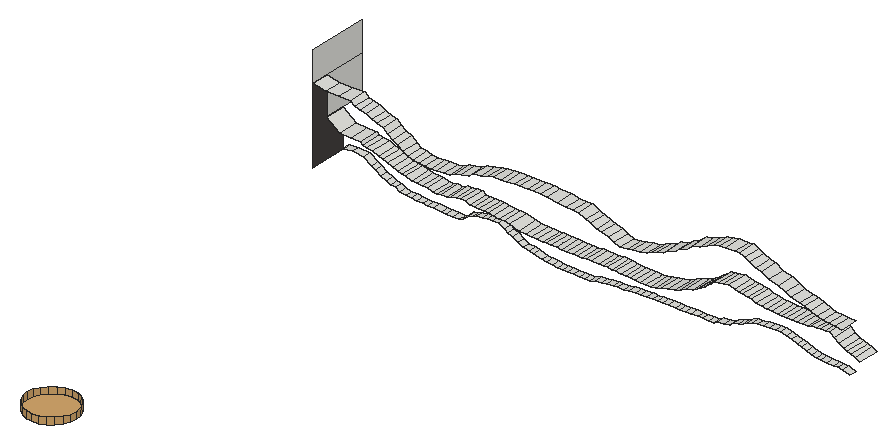
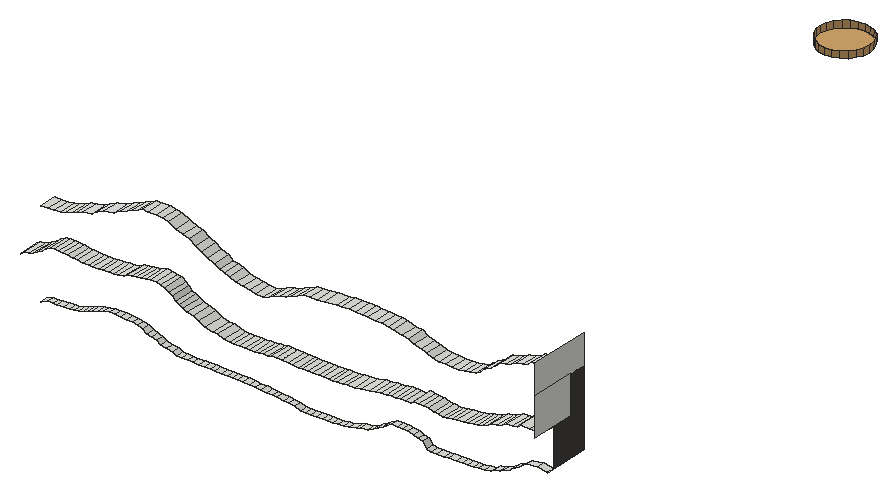
# SketchUp Ruby script. Lengths in inches.
U = 1.inch
M = Sketchup.active_model
def pt(a) = Geom::Point3d.new(a.map { |v| v * U })
def face(e, loops, mat)
  f = e.add_face(loops[0].map { |a| pt(a) })
  loops[1..].each { |l| e.add_face(l.map { |a| pt(a) }).erase! }
  f.material = f.back_material = mat if mat
  f
end
# faces: each face lists its corners as indices into pts; further lists are holes
def faces(e, pts, list, mat = nil) = list.each { |f| face(e, (f[0].is_a?(Array) ? f : [f]).map { |l| l.map { |i| pts[i] } }, mat) }
# xy, xz, yz: faces in a plane at the given z, y or x. An outline is a flat list of corners, or four numbers for a rectangle; further outlines are holes
def ring(l) = l.size == 4 ? [[l[0], l[1]], [l[2], l[1]], [l[2], l[3]], [l[0], l[3]]] : l.each_slice(2).to_a
def flat(e, list, mat, &to3) = list.each { |f| face(e, (f[0].is_a?(Array) ? f : [f]).map { |l| ring(l).map { |u, v| to3.(u, v) } }, mat) }
def xy(e, z, list, mat = nil) = flat(e, list, mat) { |x, y| [x, y, z] }
def xz(e, y, list, mat = nil) = flat(e, list, mat) { |x, z| [x, y, z] }
def yz(e, x, list, mat = nil) = flat(e, list, mat) { |y, z| [x, y, z] }
def lines(e, pts, list) = list.each { |a, b| e.add_line(pt(pts[a]), pt(pts[b])) }
# prism: a flat outline (further loops are holes) pulled along v
def prism(e, loops, v, mat = nil)
  f = face(e, loops, mat); d = Geom::Vector3d.new(v.map { |x| x * U })
  f.pushpull(f.normal.samedirection?(d) ? d.length : -d.length)
end
def box(e, o, s, mat = nil) = prism(e, [[o, [o[0] + s[0], o[1], o[2]], [o[0] + s[0], o[1] + s[1], o[2]], [o[0], o[1] + s[1], o[2]]]], [0, 0, s[2]], mat)
def at(x, y, z, deg = 0) = Geom::Transformation.translation(pt([x, y, z])) * Geom::Transformation.rotation(ORIGIN, Z_AXIS, deg.degrees)
def axes(o, x, y, z) = Geom::Transformation.new([*x, 0, *y, 0, *z, 0, *pt(o).to_a, 1])
def part(name) = M.definitions.add(name)
# library, detail: a bought-in or finely detailed component or shape, given as its bounding box
def library(name, o, s) = part(name).tap { |d| box(d.entities, o, s) }
def detail(e, o, s) = box(e.add_group.entities, o, s)
def put(e, d, t, mat = nil) = e.add_instance(d, t).tap { |i| i.material = mat if mat }
def group(e, t, mat = nil) = e.add_group.tap { |g| g.transformation = t; g.material = mat if mat }.entities
root = M.entities
M.materials.add("[Field Square Tile]").color = [211, 167, 108]
M.materials.add("[Granite Tile]1").color = [68, 65, 63]
xy(root,237.65,[[2918.33,565.74,2919.02,566.68],[2919.02,565.74,2919.64,566.68]])
xy(root,238.33,[[2927.43,565.74,2927.98,566.68],[2927.98,565.74,2928.66,566.68]])
xy(root,238.34,[[2929.34,565.74,2930.27,566.68],[2930.27,565.74,2930.76,566.68],[2930.76,565.74,2931.52,566.68],[2931.52,565.74,2932.15,566.68],[2932.15,565.74,2932.9,566.68],
  [2932.9,565.74,2933.52,566.68],[2933.52,565.74,2934.29,566.68],[2934.29,565.74,2934.91,566.68]])
xy(root,241.52,[[2889.03,561.05,2889.09,566.68]])
xy(root,241.68,[[2919.53,563.18,2920.12,565.74]])
xy(root,241.75,[[2921.88,563.18,2922.75,565.74],[2922.75,563.18,2923.37,565.74],[2923.37,563.18,2923.88,565.74]])
xy(root,250.6875,[[2909.35,492.27,2908.56,492.375,2907.82,492.68,2907.18,493.17,2906.7,493.8,2906.39,494.54,2906.29,495.33,2906.39,496.125,2906.7,496.86,2907.18,497.5,2907.82,497.98,2908.56,498.29,2909.35,498.39,2910.14,498.29,2910.88,497.98,2911.51,497.5,2912,496.86,2912.31,496.125,2912.41,495.33,2912.31,494.54,2912,493.8,2911.51,493.17,2910.88,492.68,2910.14,492.375]],"[Field Square Tile]")
xz(root,561.05,[[2889.03,241.52,2889.09,251.5]])
yz(root,2889.09,[[563.18,246.2,568.68,250.88],[561.05,250.88,568.68,254.5]])
yz(root,2889.09,[[561.05,241.52,565.74,241.52,565.74,246.2,563.18,246.2,563.18,250.88,561.05,250.88]],"[Granite Tile]1")
p = [[2919.64,565.74,237.65],[2919.64,566.68,237.65],[2920.31,566.68,237.89],[2920.31,565.74,237.89],[2914.97,565.74,237.76],[2914.97,566.68,237.76],
  [2915.68,566.68,237.71],[2915.68,565.74,237.71],[2916.29,566.68,237.68],[2916.29,565.74,237.68],[2916.89,566.68,237.67],[2916.89,565.74,237.67],
  [2917.64,566.68,237.66],[2917.64,565.74,237.66],[2918.33,566.68,237.65],[2918.33,565.74,237.65],[2913.62,565.74,237.9],[2913.62,566.68,237.9],
  [2914.28,566.68,237.82],[2914.28,565.74,237.82],[2912.68,565.74,238.21],[2912.68,566.68,238.21],[2921.07,566.68,237.94],[2921.07,565.74,237.94],
  [2921.6875,566.68,237.98],[2921.6875,565.74,237.98],[2922.54,566.68,238.1],[2922.54,565.74,238.1],[2923.09,566.68,238.13],[2923.09,565.74,238.13],
  [2923.85,566.68,238.15],[2923.85,565.74,238.15],[2912.21,565.74,238.31],[2912.21,566.68,238.31],[2924.48,566.68,238.26],[2924.48,565.74,238.26],
  [2911.3,565.74,238.43],[2911.3,566.68,238.43],[2925.23,566.68,238.28],[2925.23,565.74,238.28],[2925.86,566.68,238.3],[2925.86,565.74,238.3],
  [2926.71,566.68,238.32],[2926.71,565.74,238.32],[2927.43,566.68,238.33],[2927.43,565.74,238.33],[2928.66,565.74,238.33],[2928.66,566.68,238.33],
  [2929.34,566.68,238.34],[2929.34,565.74,238.34],[2934.91,565.74,238.34],[2934.91,566.68,238.34],[2935.42,566.68,238.59],[2935.42,565.74,238.59],
  [2910.65,565.74,238.74],[2910.65,566.68,238.74],[2950.94,565.74,238.78],[2950.94,566.68,238.78],[2951.72,566.68,238.43],[2951.72,565.74,238.43],
  [2936.24,566.68,238.72],[2936.24,565.74,238.72],[2910.07,565.74,239.11],[2910.07,566.68,239.11],[2936.93,566.68,238.86],[2936.93,565.74,238.86],
  [2900.28,565.74,238.92],[2900.28,566.68,238.92],[2901.32,566.68,238.82],[2901.32,565.74,238.82],[2901.83,566.68,238.8],[2901.83,565.74,238.8],
  [2902.7,566.68,238.79],[2902.7,565.74,238.79],[2903.44,566.68,238.77],[2903.44,565.74,238.77],[2903.97,566.68,238.9375],[2903.97,565.74,238.9375],
  [2948.22,565.74,238.875],[2948.22,566.68,238.875],[2948.97,566.68,238.83],[2948.97,565.74,238.83],[2949.73,566.68,238.8],[2949.73,565.74,238.8],
  [2950.27,566.68,238.79],[2950.27,565.74,238.79],[2898.19,565.74,238.97],[2898.19,566.68,238.97],[2898.89,566.68,238.94],[2898.89,565.74,238.94],
  [2899.59,566.68,238.93],[2899.59,565.74,238.93],[2904.53,566.68,239.55],[2904.53,565.74,239.55],[2937.44,566.68,239.18],[2937.44,565.74,239.18],
  [2947.07,565.74,239.04],[2947.07,566.68,239.04],[2947.65,566.68,238.94],[2947.65,565.74,238.94],[2896.82,565.74,239.09],[2896.82,566.68,239.09],
  [2897.51,566.68,239.03],[2897.51,565.74,239.03],[2946.41,565.74,239.29],[2946.41,566.68,239.29],[2896.04,565.74,239.19],[2896.04,566.68,239.19],
  [2909.49,565.74,239.38],[2909.49,566.68,239.38],[2895.53,565.74,239.52],[2895.53,566.68,239.52],[2938.03,566.68,239.35],[2938.03,565.74,239.35],
  [2945.83,565.74,239.53],[2945.83,566.68,239.53],[2909.03,565.74,239.71],[2909.03,566.68,239.71],[2938.59,566.68,239.52],[2938.59,565.74,239.52],
  [2894.97,565.74,239.64],[2894.97,566.68,239.64],[2939.14,566.68,239.85],[2939.14,565.74,239.85],[2945.3,565.74,239.7],[2945.3,566.68,239.7],
  [2894.52,565.74,239.86],[2894.52,566.68,239.86],[2905.11,566.68,239.69],[2905.11,565.74,239.69],[2905.66,566.68,239.88],[2905.66,565.74,239.88],
  [2908.33,565.74,240.11],[2908.33,566.68,240.11],[2944.61,565.74,239.92],[2944.61,566.68,239.92],[2939.78,566.68,240.03],[2939.78,565.74,240.03],
  [2893.73,565.74,240.2],[2893.73,566.68,240.2],[2906.39,566.68,239.99],[2906.39,565.74,239.99],[2943.98,565.74,240.11],[2943.98,566.68,240.11],
  [2906.98,566.68,240.05],[2906.98,565.74,240.05],[2907.64,566.68,240.09],[2907.64,565.74,240.09],[2940.4375,566.68,240.12],[2940.4375,565.74,240.12],
  [2941.11,566.68,240.19],[2941.11,565.74,240.19],[2943.2,565.74,240.27],[2943.2,566.68,240.27],[2893.13,565.74,240.59],[2893.13,566.68,240.59],
  [2941.875,566.68,240.23],[2941.875,565.74,240.23],[2942.58,566.68,240.25],[2942.58,565.74,240.25],[2892.59,565.74,240.85],[2892.59,566.68,240.85],
  [2891.57,565.74,241.55],[2891.57,566.68,241.55],[2925.51,563.18,241.57],[2925.51,565.74,241.57],[2926.05,565.74,241.53],[2926.05,563.18,241.53],
  [2926.67,565.74,241.51],[2926.67,563.18,241.51],[2927.22,565.74,241.49],[2927.22,563.18,241.49],[2927.92,565.74,241.48],[2927.92,563.18,241.48],
  [2928.58,565.74,241.47],[2928.58,563.18,241.47],[2929.15,565.74,241.46],[2929.15,563.18,241.46],[2929.86,565.74,241.6],[2929.86,563.18,241.6],
  [2889.09,565.74,241.52],[2889.09,566.68,241.52],[2890.3,566.68,241.69],[2890.3,565.74,241.69],[2924.9,563.18,241.66],[2924.9,565.74,241.66],
  [2930.59,565.74,241.85],[2930.59,563.18,241.85],[2915.87,563.18,241.75],[2915.87,565.74,241.75],[2916.32,565.74,241.74],[2916.32,563.18,241.74],
  [2916.87,565.74,241.72],[2916.87,563.18,241.72],[2917.5,565.74,241.71],[2917.5,563.18,241.71],[2918.13,565.74,241.7],[2918.13,563.18,241.7],
  [2918.86,565.74,241.69],[2918.86,563.18,241.69],[2919.53,565.74,241.68],[2919.53,563.18,241.68],[2920.12,563.18,241.68],[2920.12,565.74,241.68],
  [2920.61,565.74,241.67],[2920.61,563.18,241.67],[2921.3125,565.74,241.74],[2921.3125,563.18,241.74],[2921.88,565.74,241.75],[2921.88,563.18,241.75],
  [2923.88,563.18,241.75],[2923.88,565.74,241.75],[2924.37,565.74,241.67],[2924.37,563.18,241.67],[2913.68,563.18,241.89],[2913.68,565.74,241.89],
  [2914.5,565.74,241.83],[2914.5,563.18,241.83],[2915.1,565.74,241.78],[2915.1,563.18,241.78],[2931.26,565.74,241.91],[2931.26,563.18,241.91],
  [2912.91,563.18,241.96],[2912.91,565.74,241.96],[2932.16,565.74,242.1],[2932.16,563.18,242.1],[2911.74,563.18,242.24],[2911.74,565.74,242.24],
  [2932.93,565.74,242.46],[2932.93,563.18,242.46],[2911.07,563.18,242.34],[2911.07,565.74,242.34],[2954.54,563.18,242.51],[2954.54,565.74,242.51],
  [2955.05,565.74,242.21],[2955.05,563.18,242.21],[2910.41,563.18,242.38],[2910.41,565.74,242.38],[2909.75,563.18,242.48],[2909.75,565.74,242.48],
  [2901.57,563.18,242.68],[2901.57,565.74,242.68],[2902.24,565.74,242.51],[2902.24,563.18,242.51],[2902.76,565.74,242.46],[2902.76,563.18,242.46],
  [2903.3,565.74,242.58],[2903.3,563.18,242.58],[2909.11,563.18,242.57],[2909.11,565.74,242.57],[2933.63,565.74,242.78],[2933.63,563.18,242.78],
  [2953.95,563.18,242.68],[2953.95,565.74,242.68],[2903.93,565.74,242.57],[2903.93,563.18,242.57],[2904.56,565.74,242.81],[2904.56,563.18,242.81],
  [2906.33,563.18,242.92],[2906.33,565.74,242.92],[2906.76,565.74,242.625],[2906.76,563.18,242.625],[2907.37,565.74,242.65],[2907.37,563.18,242.65],
  [2907.92,565.74,242.62],[2907.92,563.18,242.62],[2908.55,565.74,242.58],[2908.55,563.18,242.58],[2900.22,563.18,242.78],[2900.22,565.74,242.78],
  [2901.03,565.74,242.73],[2901.03,563.18,242.73],[2953.45,563.18,242.875],[2953.45,565.74,242.875],[2898.92,563.18,243.06],[2898.92,565.74,243.06],
  [2899.64,565.74,242.85],[2899.64,563.18,242.85],[2905.13,565.74,242.86],[2905.13,563.18,242.86],[2934.4,565.74,242.97],[2934.4,563.18,242.97],
  [2905.69,565.74,242.89],[2905.69,563.18,242.89],[2953.06,563.18,243.09],[2953.06,565.74,243.09],[2934.93,565.74,243.23],[2934.93,563.18,243.23],
  [2897.85,563.18,243.3],[2897.85,565.74,243.3],[2898.4375,565.74,243.14],[2898.4375,563.18,243.14],[2952.45,563.18,243.43],[2952.45,565.74,243.43],
  [2935.33,565.74,243.48],[2935.33,563.18,243.48],[2897.21,563.18,243.48],[2897.21,565.74,243.48],[2951.91,563.18,243.8],[2951.91,565.74,243.8],
  [2896.69,563.18,243.79],[2896.69,565.74,243.79],[2935.85,565.74,243.72],[2935.85,563.18,243.72],[2936.1875,565.74,244.12],[2936.1875,563.18,244.12],
  [2896.03,563.18,243.95],[2896.03,565.74,243.95],[2951.31,563.18,244.18],[2951.31,565.74,244.18],[2895.51,563.18,244.11],[2895.51,565.74,244.11],
  [2944.13,563.18,243.99],[2944.13,565.74,243.99],[2944.85,565.74,243.95],[2944.85,563.18,243.95],[2945.35,565.74,243.93],[2945.35,563.18,243.93],
  [2946.04,565.74,243.91],[2946.04,563.18,243.91],[2946.61,565.74,243.89],[2946.61,563.18,243.89],[2947.31,565.74,243.88],[2947.31,563.18,243.88],
  [2947.96,565.74,243.94],[2947.96,563.18,243.94],[2948.6,565.74,243.95],[2948.6,563.18,243.95],[2949.16,565.74,244.1],[2949.16,563.18,244.1],
  [2942.95,563.18,244.11],[2942.95,565.74,244.11],[2943.51,565.74,244.04],[2943.51,563.18,244.04],[2894.84,563.18,244.41],[2894.84,565.74,244.41],
  [2936.66,565.74,244.39],[2936.66,563.18,244.39],[2942.2,563.18,244.25],[2942.2,565.74,244.25],[2949.79,565.74,244.13],[2949.79,563.18,244.13],
  [2950.27,565.74,244.15],[2950.27,563.18,244.15],[2950.79,565.74,244.17],[2950.79,563.18,244.17],[2941.74,563.18,244.51],[2941.74,565.74,244.51],
  [2894.08,563.18,244.54],[2894.08,565.74,244.54],[2937.14,565.74,244.73],[2937.14,563.18,244.73],[2893.52,563.18,244.61],[2893.52,565.74,244.61],
  [2940.59,563.18,244.67],[2940.59,565.74,244.67],[2941.2,565.74,244.55],[2941.2,563.18,244.55],[2893.3,563.18,244.92],[2893.3,565.74,244.92],
  [2937.625,565.74,244.87],[2937.625,563.18,244.87],[2939.54,563.18,244.81],[2939.54,565.74,244.81],[2940.11,565.74,244.7],[2940.11,563.18,244.7],
  [2938.89,563.18,245.01],[2938.89,565.74,245.01],[2890.66,563.18,244.96],[2890.66,565.74,244.96],[2892.05,565.74,244.9375],[2892.05,563.18,244.9375],
  [2938.21,565.74,244.95],[2938.21,563.18,244.95],[2889.09,563.18,246.2],[2889.09,565.74,246.2],[2926.34,561.05,246.35],[2926.34,563.18,246.35],
  [2927.11,563.18,246.05],[2927.11,561.05,246.05],[2928.01,563.18,246.13],[2928.01,561.05,246.13],[2928.72,563.18,246.29],[2928.72,561.05,246.29],
  [2929.52,563.18,246.41],[2929.52,561.05,246.41],[2925.73,561.05,246.66],[2925.73,563.18,246.66],[2930.43,563.18,246.55],[2930.43,561.05,246.55],
  [2902.15,561.05,246.62],[2902.15,563.18,246.62],[2902.89,563.18,246.54],[2902.89,561.05,246.54],[2903.67,563.18,246.51],[2903.67,561.05,246.51],
  [2904.45,563.18,246.58],[2904.45,561.05,246.58],[2953.64,561.05,246.59],[2953.64,563.18,246.59],[2954.53,563.18,246.55],[2954.53,561.05,246.55],
  [2901.49,561.05,246.73],[2901.49,563.18,246.73],[2905.25,563.18,246.59],[2905.25,561.05,246.59],[2906.05,563.18,246.69],[2906.05,561.05,246.69],
  [2931.16,563.18,246.92],[2931.16,561.05,246.92],[2952.93,561.05,246.66],[2952.93,563.18,246.66],[2900.77,561.05,246.88],[2900.77,563.18,246.88],
  [2906.76,563.18,247.03],[2906.76,561.05,247.03],[2924.875,561.05,246.94],[2924.875,563.18,246.94],[2952.14,561.05,246.75],[2952.14,563.18,246.75],
  [2951.45,561.05,246.95],[2951.45,563.18,246.95],[2900.22,561.05,247.25],[2900.22,563.18,247.25],[2924.19,561.05,247.08],[2924.19,563.18,247.08],
  [2931.77,563.18,247.12],[2931.77,561.05,247.12],[2907.45,563.18,247.2],[2907.45,561.05,247.2],[2950.64,561.05,247.25],[2950.64,563.18,247.25],
  [2923.51,561.05,247.46],[2923.51,563.18,247.46],[2932.45,563.18,247.31],[2932.45,561.05,247.31],[2908.42,563.18,247.39],[2908.42,561.05,247.39],
  [2949.96,561.05,247.53],[2949.96,563.18,247.53],[2899.58,561.05,247.72],[2899.58,563.18,247.72],[2933.02,563.18,247.71],[2933.02,561.05,247.71],
  [2909.05,563.18,247.78],[2909.05,561.05,247.78],[2922.88,561.05,247.66],[2922.88,563.18,247.66],[2949.38,561.05,247.66],[2949.38,563.18,247.66],
  [2898.93,561.05,248.07],[2898.93,563.18,248.07],[2922.04,561.05,248.08],[2922.04,563.18,248.08],[2933.95,563.18,248.03],[2933.95,561.05,248.03],
  [2948.25,561.05,247.9],[2948.25,563.18,247.9],[2909.83,563.18,247.89],[2909.83,561.05,247.89],[2910.83,563.18,248.18],[2910.83,561.05,248.18],
  [2947.65,561.05,248.26],[2947.65,563.18,248.26],[2934.66,563.18,248.46],[2934.66,561.05,248.46],[2898.3,561.05,248.51],[2898.3,563.18,248.51],
  [2920.42,561.05,248.15],[2920.42,563.18,248.15],[2921.24,563.18,248.11],[2921.24,561.05,248.11],[2911.47,563.18,248.29],[2911.47,561.05,248.29],
  [2919.39,561.05,248.28],[2919.39,563.18,248.28],[2912.36,563.18,248.35],[2912.36,561.05,248.35],[2917.99,561.05,248.39],[2917.99,563.18,248.39],
  [2946.74,561.05,248.69],[2946.74,563.18,248.69],[2913.09,563.18,248.4],[2913.09,561.05,248.4],[2914.08,563.18,248.4375],[2914.08,561.05,248.4375],
  [2914.74,563.18,248.46],[2914.74,561.05,248.46],[2917.26,561.05,248.49],[2917.26,563.18,248.49],[2897.81,561.05,249.01],[2897.81,563.18,249.01],
  [2915.63,563.18,248.47],[2915.63,561.05,248.47],[2916.37,563.18,248.48],[2916.37,561.05,248.48],[2935.44,563.18,248.82],[2935.44,561.05,248.82],
  [2945.52,561.05,248.95],[2945.52,563.18,248.95],[2936.16,563.18,249.37],[2936.16,561.05,249.37],[2944.63,561.05,249.46],[2944.63,563.18,249.46],
  [2897.04,561.05,249.2],[2897.04,563.18,249.2],[2896.37,561.05,249.41],[2896.37,563.18,249.41],[2895.7,561.05,249.8],[2895.7,563.18,249.8],
  [2936.95,563.18,249.5625],[2936.95,561.05,249.5625],[2943.87,561.05,249.68],[2943.87,563.18,249.68],[2937.85,563.18,249.9],[2937.85,561.05,249.9],
  [2943.21,561.05,250.0625],[2943.21,563.18,250.0625],[2894.9,561.05,249.97],[2894.9,563.18,249.97],[2938.77,563.18,250.35],[2938.77,561.05,250.35],
  [2894.29,561.05,250.15],[2894.29,563.18,250.15],[2893.76,561.05,250.55],[2893.76,563.18,250.55],[2942.52,561.05,250.32],[2942.52,563.18,250.32],
  [2939.43,563.18,250.49],[2939.43,561.05,250.49],[2941.9,561.05,250.61],[2941.9,563.18,250.61],[2889.09,561.05,250.88],[2889.09,563.18,250.88],
  [2890.68,563.18,250.53],[2890.68,561.05,250.53],[2892.3,563.18,250.54],[2892.3,561.05,250.54],[2940.24,563.18,250.6],[2940.24,561.05,250.6],
  [2941.26,563.18,250.58],[2941.26,561.05,250.58],[2909.35,492.27,251.5],[2908.56,492.375,251.5],[2908.56,492.375,250.6875],[2909.35,492.27,250.6875],
  [2910.14,492.375,251.5],[2910.14,492.375,250.6875],[2907.82,492.68,251.5],[2907.82,492.68,250.6875],[2910.88,492.68,251.5],[2910.88,492.68,250.6875],
  [2907.18,493.17,251.5],[2907.18,493.17,250.6875],[2911.51,493.17,251.5],[2911.51,493.17,250.6875],[2906.7,493.8,251.5],[2906.7,493.8,250.6875],
  [2912,493.8,251.5],[2912,493.8,250.6875],[2906.39,494.54,251.5],[2906.39,494.54,250.6875],[2912.31,494.54,251.5],[2912.31,494.54,250.6875],
  [2906.29,495.33,251.5],[2906.29,495.33,250.6875],[2912.41,495.33,251.5],[2912.41,495.33,250.6875],[2906.39,496.125,251.5],[2906.39,496.125,250.6875],
  [2912.31,496.125,251.5],[2912.31,496.125,250.6875],[2906.7,496.86,251.5],[2906.7,496.86,250.6875],[2912,496.86,251.5],[2912,496.86,250.6875],
  [2907.18,497.5,251.5],[2907.18,497.5,250.6875],[2911.51,497.5,251.5],[2911.51,497.5,250.6875],[2907.82,497.98,251.5],[2907.82,497.98,250.6875],
  [2910.88,497.98,251.5],[2910.88,497.98,250.6875],[2908.56,498.29,251.5],[2908.56,498.29,250.6875],[2910.14,498.29,251.5],[2910.14,498.29,250.6875],
  [2909.35,498.39,251.5],[2909.35,498.39,250.6875]]
faces(root,p,[[0,1,2,3],[4,5,6,7],[7,6,8,9],[9,8,10,11],[11,10,12,13],[13,12,14,15],[16,17,18,19],[19,18,5,4],
  [20,21,17,16],[3,2,22,23],[23,22,24,25],[25,24,26,27],[27,26,28,29],[29,28,30,31],[32,33,21,20],[31,30,34,35],
  [36,37,33,32],[35,34,38,39],[39,38,40,41],[41,40,42,43],[43,42,44,45],[46,47,48,49],[50,51,52,53],[54,55,37,36],
  [56,57,58,59],[53,52,60,61],[62,63,55,54],[61,60,64,65],[66,67,68,69],[69,68,70,71],[71,70,72,73],[73,72,74,75],
  [75,74,76,77],[78,79,80,81],[81,80,82,83],[83,82,84,85],[85,84,57,56],[86,87,88,89],[89,88,90,91],[91,90,67,66],
  [77,76,92,93],[65,64,94,95],[96,97,98,99],[99,98,79,78],[100,101,102,103],[103,102,87,86],[104,105,97,96],[106,107,101,100],
  [108,109,63,62],[110,111,107,106],[95,94,112,113],[114,115,105,104],[116,117,109,108],[113,112,118,119],[120,121,111,110],[119,118,122,123],
  [124,125,115,114],[126,127,121,120],[93,92,128,129],[129,128,130,131],[132,133,117,116],[134,135,125,124],[123,122,136,137],[138,139,127,126],
  [131,130,140,141],[142,143,135,134],[141,140,144,145],[145,144,146,147],[137,136,148,149],[147,146,133,132],[149,148,150,151],[152,153,143,142],
  [154,155,139,138],[151,150,156,157],[157,156,158,159],[159,158,153,152],[160,161,155,154],[162,163,161,160],[164,165,166,167],[167,166,168,169],
  [169,168,170,171],[171,170,172,173],[173,172,174,175],[175,174,176,177],[177,176,178,179],[180,181,182,183],[184,185,165,164],[179,178,186,187],
  [183,182,163,162],[188,189,190,191],[191,190,192,193],[193,192,194,195],[195,194,196,197],[197,196,198,199],[199,198,200,201],[202,203,204,205],
  [205,204,206,207],[207,206,208,209],[210,211,212,213],[213,212,185,184],[214,215,216,217],[217,216,218,219],[219,218,189,188],[187,186,220,221],
  [222,223,215,214],[221,220,224,225],[226,227,223,222],[225,224,228,229],[230,231,227,226],[232,233,234,235],[236,237,231,230],[238,239,237,236],
  [240,241,242,243],[243,242,244,245],[245,244,246,247],[248,249,239,238],[229,228,250,251],[252,253,233,232],[247,246,254,255],[255,254,256,257],
  [258,259,260,261],[261,260,262,263],[263,262,264,265],[265,264,266,267],[267,266,249,248],[268,269,270,271],[271,270,241,240],[272,273,253,252],
  [274,275,276,277],[277,276,269,268],[257,256,278,279],[251,250,280,281],[279,278,282,283],[283,282,259,258],[284,285,273,272],[281,280,286,287],
  [288,289,290,291],[291,290,275,274],[292,293,285,284],[287,286,294,295],[296,297,289,288],[298,299,293,292],[300,301,297,296],[295,294,302,303],
  [303,302,304,305],[306,307,301,300],[308,309,299,298],[310,311,307,306],[312,313,314,315],[315,314,316,317],[317,316,318,319],[319,318,320,321],
  [321,320,322,323],[323,322,324,325],[325,324,326,327],[327,326,328,329],[330,331,332,333],[333,332,313,312],[334,335,311,310],[305,304,336,337],
  [338,339,331,330],[329,328,340,341],[341,340,342,343],[343,342,344,345],[345,344,309,308],[346,347,339,338],[348,349,335,334],[337,336,350,351],
  [352,353,349,348],[354,355,356,357],[357,356,347,346],[358,359,353,352],[351,350,360,361],[362,363,364,365],[365,364,355,354],[366,367,363,362],
  [368,369,370,371],[371,370,359,358],[361,360,372,373],[373,372,367,366],[374,375,369,368],[376,377,378,379],[379,378,380,381],[381,380,382,383],
  [383,382,384,385],[386,387,377,376],[385,384,388,389],[390,391,392,393],[393,392,394,395],[395,394,396,397],[398,399,400,401],[402,403,391,390],
  [397,396,404,405],[405,404,406,407],[389,388,408,409],[410,411,399,398],[412,413,403,402],[407,406,414,415],[416,417,387,386],[418,419,411,410],
  [420,421,419,418],[422,423,413,412],[424,425,417,416],[409,408,426,427],[415,414,428,429],[430,431,421,420],[432,433,425,424],[427,426,434,435],
  [429,428,436,437],[438,439,431,430],[440,441,423,422],[435,434,442,443],[437,436,444,445],[446,447,433,432],[448,449,439,438],[450,451,441,440],
  [452,453,447,446],[443,442,454,455],[456,457,449,448],[445,444,458,459],[459,458,460,461],[462,463,457,456],[455,454,464,465],[466,467,451,450],
  [468,469,470,471],[471,470,453,452],[461,460,472,473],[474,475,469,468],[473,472,476,477],[478,479,475,474],[480,481,463,462],[477,476,482,483],
  [483,482,484,485],[485,484,486,487],[488,489,479,478],[490,491,467,466],[487,486,492,493],[493,492,494,495],[495,494,489,488],[465,464,496,497],
  [498,499,481,480],[497,496,500,501],[502,503,499,498],[504,505,491,490],[506,507,505,504],[508,509,507,506],[501,500,510,511],[512,513,503,502],
  [511,510,514,515],[516,517,513,512],[518,519,509,508],[515,514,520,521],[522,523,519,518],[524,525,523,522],[526,527,517,516],[521,520,528,529],
  [530,531,527,526],[532,533,534,535],[535,534,536,537],[537,536,525,524],[529,528,538,539],[539,538,540,541],[541,540,531,530]])
faces(root,p,[[542,543,544,545],[546,542,545,547],[543,548,549,544],[550,546,547,551],[548,552,553,549],[554,550,551,555],[552,556,557,553],[558,554,555,559],
  [556,560,561,557],[562,558,559,563],[560,564,565,561],[566,562,563,567],[564,568,569,565],[570,566,567,571],[568,572,573,569],[574,570,571,575],
  [572,576,577,573],[578,574,575,579],[576,580,581,577],[582,578,579,583],[580,584,585,581],[586,582,583,587],[584,588,589,585],[588,586,587,589]],"[Field Square Tile]")
